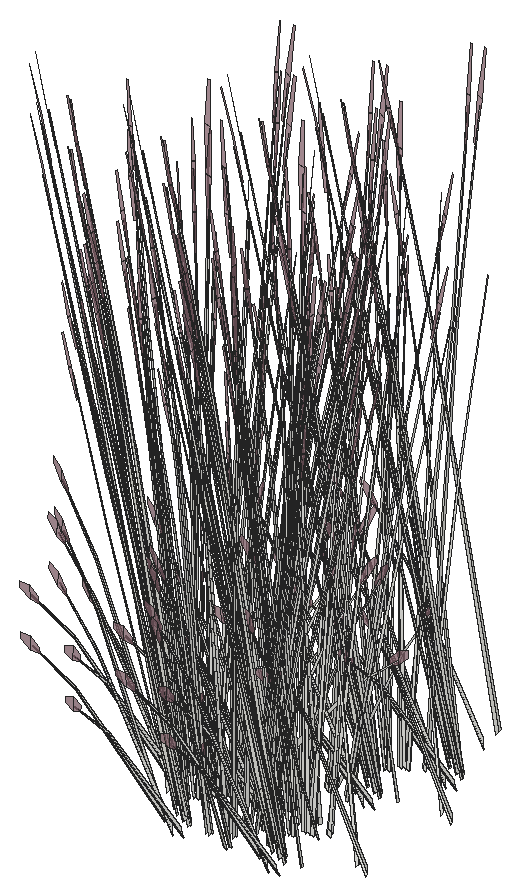
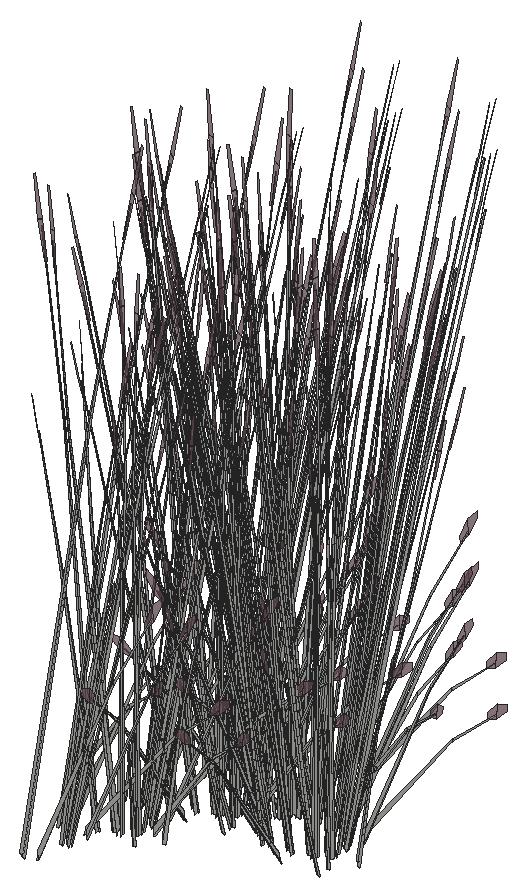
# SketchUp Ruby script. Lengths in inches.
U = 1.inch
M = Sketchup.active_model
def pt(a) = Geom::Point3d.new(a.map { |v| v * U })
def face(e, loops, mat)
  f = e.add_face(loops[0].map { |a| pt(a) })
  loops[1..].each { |l| e.add_face(l.map { |a| pt(a) }).erase! }
  f.material = f.back_material = mat if mat
  f
end
# faces: each face lists its corners as indices into pts; further lists are holes
def faces(e, pts, list, mat = nil) = list.each { |f| face(e, (f[0].is_a?(Array) ? f : [f]).map { |l| l.map { |i| pts[i] } }, mat) }
# xy, xz, yz: faces in a plane at the given z, y or x. An outline is a flat list of corners, or four numbers for a rectangle; further outlines are holes
def ring(l) = l.size == 4 ? [[l[0], l[1]], [l[2], l[1]], [l[2], l[3]], [l[0], l[3]]] : l.each_slice(2).to_a
def flat(e, list, mat, &to3) = list.each { |f| face(e, (f[0].is_a?(Array) ? f : [f]).map { |l| ring(l).map { |u, v| to3.(u, v) } }, mat) }
def xy(e, z, list, mat = nil) = flat(e, list, mat) { |x, y| [x, y, z] }
def xz(e, y, list, mat = nil) = flat(e, list, mat) { |x, z| [x, y, z] }
def yz(e, x, list, mat = nil) = flat(e, list, mat) { |y, z| [x, y, z] }
def lines(e, pts, list) = list.each { |a, b| e.add_line(pt(pts[a]), pt(pts[b])) }
# prism: a flat outline (further loops are holes) pulled along v
def prism(e, loops, v, mat = nil)
  f = face(e, loops, mat); d = Geom::Vector3d.new(v.map { |x| x * U })
  f.pushpull(f.normal.samedirection?(d) ? d.length : -d.length)
end
def box(e, o, s, mat = nil) = prism(e, [[o, [o[0] + s[0], o[1], o[2]], [o[0] + s[0], o[1] + s[1], o[2]], [o[0], o[1] + s[1], o[2]]]], [0, 0, s[2]], mat)
def at(x, y, z, deg = 0) = Geom::Transformation.translation(pt([x, y, z])) * Geom::Transformation.rotation(ORIGIN, Z_AXIS, deg.degrees)
def axes(o, x, y, z) = Geom::Transformation.new([*x, 0, *y, 0, *z, 0, *pt(o).to_a, 1])
def part(name) = M.definitions.add(name)
# library, detail: a bought-in or finely detailed component or shape, given as its bounding box
def library(name, o, s) = part(name).tap { |d| box(d.entities, o, s) }
def detail(e, o, s) = box(e.add_group.entities, o, s)
def put(e, d, t, mat = nil) = e.add_instance(d, t).tap { |i| i.material = mat if mat }
def group(e, t, mat = nil) = e.add_group.tap { |g| g.transformation = t; g.material = mat if mat }.entities
root = M.entities
M.materials.add("LightPink_Translucent").color = [144, 107, 117]
M.materials["LightPink_Translucent"].alpha = 0.75
c1 = part("blade")
p = [[2.15,0.21,22],[0,0.17,0],[0.09,0.45,0],[2.18,0.31,22],[2.29,0.31,22],[0.38,0.45,0],
  [2.48,0.24,33],[2.49,0.24,33],[2.48,0.22,33]]
faces(c1.entities,p,[[0,1,2,3],[4,5,2,3],[6,3,4,7],[8,0,3,6]])
c2 = part("seeds")
p = [[0.3,-0.1,1.38],[-0.01,-0.03,1.59],[-0.01,-0.03,0.03],[0.14,-0.07,-0.07],[0.29,-0.03,3],[0.15,0.01,3.11]]
faces(c2.entities,p,[[0,1,2,3],[1,0,4,5]],"LightPink_Translucent")
c3 = part("blade with seeds")
put(c3.entities,c1,at(0,0,0))
put(c3.entities,c2,axes([2.4,0.25,30.99],[1.5799,-0.05474,1.17369],[-0.12525,1.92788,0.29478],[-0.07173,-0.02425,1.56792]))
put(root,c3,axes([321.88,20.77,52.16],[0.06444,0.01048,1.56736],[0.19934,0.34525,-0.1481],[-0.13191,0.09062,0.27737]))
put(root,c3,axes([323.19,18.85,52.16],[0.03743,0.039,1.56736],[-0.18045,0.35054,-0.1481],[-0.18276,0.00254,0.27737]))
put(root,c3,axes([323.61,18.62,52.17],[-0.10864,-0.00276,1.54581],[-0.34587,0.27582,-0.24447],[-0.18454,-0.05636,0.12397]))
put(root,c3,axes([323.16,20.14,52.18],[0.14265,-0.35629,0.42415],[0.46898,0.12183,0.34973],[-0.18443,0.02141,0.87768]))
put(root,c3,axes([323.13,20.05,52.18],[-0.18545,-0.26643,0.05682],[0.33817,-0.13041,0.44729],[-0.14907,0.02573,0.68204]))
put(root,c3,axes([323.28,21.03,52.18],[-0.12522,-0.35963,0.42415],[0.49122,-0.06241,0.34973],[-0.14477,0.08458,0.87768]))
put(root,c3,axes([323.53,19.24,52.5],[0.41698,-0.28837,0.47505],[0.35962,0.30624,0.3917],[-0.19563,-0.05319,0.983]))
put(root,c3,axes([323.18,20.96,52.18],[-0.34663,-0.16434,0.05682],[0.20181,-0.23402,0.44729],[-0.11113,0.07566,0.68204]))
put(root,c3,axes([323.51,20.15,52.46],[0.41962,0.10901,0.31292],[-0.12239,0.31802,-0.40398],[-0.16894,0.02916,0.77298]))
put(root,c3,axes([323.72,19.24,52.18],[0.02542,-0.29714,0.05682],[0.38391,0.00815,0.44729],[-0.14706,-0.03109,0.68204]))
put(root,c3,axes([322.81,21.78,52.17],[-0.01255,0.07733,1.54581],[0.35618,0.269,-0.24447],[-0.09325,0.12721,0.12397]))
put(root,c3,axes([324.9,18.72,52.8],[-0.33698,0.3746,-0.12034],[-0.48801,-0.21581,-0.66795],[-0.16964,-0.10584,1.01494]))
put(root,c3,axes([323.98,19.46,52.46],[0.28729,0.24465,0.31292],[-0.32804,0.23159,-0.40398],[-0.16667,-0.03524,0.77298]))
put(root,c3,axes([322.58,21.82,52.99],[0.44556,0.1043,-0.05733],[-0.13706,0.32103,-0.25992],[-0.07288,0.04874,0.85731]))
put(root,c3,axes([323.58,20.91,52.46],[0.43951,-0.05584,0.31292],[0.11606,0.31924,-0.40398],[-0.12595,0.08575,0.77298]))
put(root,c3,axes([324.77,17.83,52.16],[-0.00942,0.04684,1.56736],[-0.46458,0.16998,-0.1481],[-0.13671,-0.08689,0.27737]))
put(root,c3,axes([325.82,16.68,52.17],[-0.08245,0.05073,1.54581],[0.00701,0.37067,-0.24447],[-0.18899,0.0482,0.12397]))
put(root,c3,axes([323.99,21.76,52.18],[-0.35954,-0.26661,0.42415],[0.38183,-0.22994,0.34973],[-0.06632,0.12508,0.87768]))
put(root,c3,axes([323.86,21.73,52.18],[-0.41493,-0.01821,0.05682],[0.01138,-0.27493,0.44729],[-0.04342,0.10531,0.68204]))
put(root,c3,axes([324.91,17.06,52.16],[0.06444,0.01048,1.56736],[0.19934,0.34525,-0.1481],[-0.13191,0.09062,0.27737]))
put(root,c3,axes([324.87,19.04,52.46],[0.07798,0.31474,0.31292],[-0.44579,0.08311,-0.40398],[-0.11974,-0.09019,0.77298]))
put(root,c3,axes([322.77,22.57,52.16],[0.05728,-0.02359,1.56736],[0.47345,0.15692,-0.1481],[-0.01113,0.13066,0.27737]))
put(root,c3,axes([326.21,15.14,52.16],[0.03743,0.039,1.56736],[-0.18045,0.35054,-0.1481],[-0.18276,0.00254,0.27737]))
put(root,c3,axes([326.63,14.91,52.17],[-0.10864,-0.00276,1.54581],[-0.34587,0.27582,-0.24447],[-0.18454,-0.05636,0.12397]))
put(root,c3,axes([324.67,18.67,52.5],[0.56246,-0.10044,0.47505],[0.09762,0.39398,0.3917],[-0.13228,-0.11611,0.983]))
put(root,c3,axes([326.18,16.43,52.18],[0.14265,-0.35629,0.42415],[0.46898,0.12183,0.34973],[-0.18443,0.02141,0.87768]))
put(root,c3,axes([326.15,16.34,52.18],[-0.18545,-0.26643,0.05682],[0.33817,-0.13041,0.44729],[-0.14907,0.02573,0.68204]))
put(root,c3,axes([324.8,18.75,52.18],[0.22948,-0.24822,0.05682],[0.32679,0.14452,0.44729],[-0.10565,-0.07958,0.68204]))
put(root,c3,axes([325.3,18.01,52.17],[-0.07723,-0.05479,1.54581],[-0.51538,0.03473,-0.24447],[-0.08225,-0.13104,0.12397]))
put(root,c3,axes([326.3,17.32,52.18],[-0.12522,-0.35963,0.42415],[0.49122,-0.06241,0.34973],[-0.14477,0.08458,0.87768]))
put(root,c3,axes([326.55,15.53,52.5],[0.41698,-0.28837,0.47505],[0.35962,0.30624,0.3917],[-0.19563,-0.05319,0.983]))
put(root,c3,axes([326.2,17.25,52.18],[-0.34663,-0.16434,0.05682],[0.20181,-0.23402,0.44729],[-0.11113,0.07566,0.68204]))
put(root,c3,axes([324.17,21.55,52.46],[0.34164,-0.20573,0.31292],[0.3234,0.23491,-0.40398],[-0.04921,0.11936,0.77298]))
put(root,c3,axes([326.53,16.4375,52.46],[0.41962,0.10901,0.31292],[-0.12239,0.31802,-0.40398],[-0.16894,0.02916,0.77298]))
put(root,c3,axes([323.95,21.6,52.77],[0.55492,0.01936,-0.11927],[-0.01517,0.36657,-0.66198],[-0.03855,0.14118,1.00587]))
put(root,c3,axes([326.74,15.53,52.18],[0.02542,-0.29714,0.05682],[0.38391,0.00815,0.44729],[-0.14706,-0.03109,0.68204]))
put(root,c3,axes([325.84,18.07,52.17],[-0.01255,0.07733,1.54581],[0.35618,0.269,-0.24447],[-0.09325,0.12721,0.12397]))
put(root,c3,axes([327.92,15.02,52.8],[-0.33698,0.3746,-0.12034],[-0.48801,-0.21581,-0.66795],[-0.16964,-0.10584,1.01494]))
put(root,c3,axes([327,15.75,52.46],[0.28729,0.24465,0.31292],[-0.32804,0.23159,-0.40398],[-0.16667,-0.03524,0.77298]))
put(root,c3,axes([325.93,18.99,52.46],[-0.15222,0.30049,0.31292],[-0.44409,-0.08764,-0.40398],[-0.04072,-0.12098,0.77298]))
put(root,c3,axes([325.6,18.11,52.99],[0.44556,0.1043,-0.05733],[-0.13706,0.32103,-0.25992],[-0.07288,0.04874,0.85731]))
put(root,c3,axes([326.6,17.2,52.46],[0.43951,-0.05584,0.31292],[0.11606,0.31924,-0.40398],[-0.12595,0.08575,0.77298]))
put(root,c3,axes([325.125,22.13,52.47],[-0.49753,-0.10215,0.47081],[0.17013,-0.33585,0.3882],[0.0299,0.13207,0.97422]))
put(root,c3,axes([324.99,22.16,52.18],[-0.37205,0.1328,0.05682],[-0.18211,-0.24217,0.44729],[0.03593,0.10675,0.68204]))
put(root,c3,axes([328.62,20.09,52.17],[-0.08245,0.05073,1.54581],[0.00701,0.37067,-0.24447],[-0.18899,0.0482,0.12397]))
put(root,c3,axes([327.79,14.125,52.16],[-0.00942,0.04684,1.56736],[-0.46458,0.16998,-0.1481],[-0.13671,-0.08689,0.27737]))
put(root,c3,axes([327.02,18.05,52.18],[-0.35954,-0.26661,0.42415],[0.38183,-0.22994,0.34973],[-0.06632,0.12508,0.87768]))
put(root,c3,axes([327.7,20.46,52.16],[0.06444,0.01048,1.56736],[0.19934,0.34525,-0.1481],[-0.13191,0.09062,0.27737]))
put(root,c3,axes([326.88,18.02,52.18],[-0.41493,-0.01821,0.05682],[0.01138,-0.27493,0.44729],[-0.04342,0.10531,0.68204]))
put(root,c3,axes([329.01,18.54,52.16],[0.03743,0.039,1.56736],[-0.18045,0.35054,-0.1481],[-0.18276,0.00254,0.27737]))
put(root,c3,axes([327.89,15.33,52.46],[0.07798,0.31474,0.31292],[-0.44579,0.08311,-0.40398],[-0.11974,-0.09019,0.77298]))
put(root,c3,axes([325.8,18.86,52.16],[0.05728,-0.02359,1.56736],[0.47345,0.15692,-0.1481],[-0.01113,0.13066,0.27737]))
put(root,c3,axes([329.43,18.31,52.17],[-0.10864,-0.00276,1.54581],[-0.34587,0.27582,-0.24447],[-0.18454,-0.05636,0.12397]))
put(root,c3,axes([328.98,19.83,52.18],[0.14265,-0.35629,0.42415],[0.46898,0.12183,0.34973],[-0.18443,0.02141,0.87768]))
put(root,c3,axes([326.07,18.71,52.18],[0.37205,-0.1328,0.05682],[0.18211,0.24217,0.44729],[-0.03593,-0.10675,0.68204]))
put(root,c3,axes([324.86,22.73,52.17],[0.064,0.06292,1.54581],[0.51651,0.02472,-0.24447],[0.05194,0.13877,0.12397]))
put(root,c3,axes([328.95,19.74,52.18],[-0.18545,-0.26643,0.05682],[0.33817,-0.13041,0.44729],[-0.14907,0.02573,0.68204]))
put(root,c3,axes([325.94,18.74,52.18],[0.49753,0.10215,0.42415],[-0.17013,0.33585,0.34973],[-0.0299,-0.13207,0.87768]))
put(root,c3,axes([327.69,14.96,52.5],[0.56246,-0.10044,0.47505],[0.09762,0.39398,0.3917],[-0.13228,-0.11611,0.983]))
put(root,c3,axes([325.13,21.88,52.46],[0.15222,-0.30049,0.31292],[0.44409,0.08764,-0.40398],[0.04072,0.12098,0.77298]))
put(root,c3,axes([327.82,15.04,52.18],[0.22948,-0.24822,0.05682],[0.32679,0.14452,0.44729],[-0.10565,-0.07958,0.68204]))
put(root,c3,axes([329.09,20.72,52.18],[-0.12522,-0.35963,0.42415],[0.49122,-0.06241,0.34973],[-0.14477,0.08458,0.87768]))
put(root,c3,axes([329.35,18.93,52.5],[0.41698,-0.28837,0.47505],[0.35962,0.30624,0.3917],[-0.19563,-0.05319,0.983]))
put(root,c3,axes([329,20.65,52.18],[-0.34663,-0.16434,0.05682],[0.20181,-0.23402,0.44729],[-0.11113,0.07566,0.68204]))
put(root,c3,axes([328.32,14.3,52.17],[-0.07723,-0.05479,1.54581],[-0.51538,0.03473,-0.24447],[-0.08225,-0.13104,0.12397]))
put(root,c3,axes([325.73,22.96,52.99],[0.34892,-0.22417,-0.05733],[0.3197,0.24551,-0.25992],[0.02251,0.06957,0.85731]))
put(root,c3,axes([329.33,19.84,52.46],[0.41962,0.10901,0.31292],[-0.12239,0.31802,-0.40398],[-0.16894,0.02916,0.77298]))
put(root,c3,axes([327.19,17.84,52.46],[0.34164,-0.20573,0.31292],[0.3234,0.23491,-0.40398],[-0.04921,0.11936,0.77298]))
put(root,c3,axes([329.54,18.93,52.18],[0.02542,-0.29714,0.05682],[0.38391,0.00815,0.44729],[-0.14706,-0.03109,0.68204]))
put(root,c3,axes([327.5,18.41,52.16],[-0.05128,0.02985,1.56736],[-0.5024,-0.1007,-0.1481],[-0.01819,-0.13025,0.27737]))
put(root,c3,axes([328.63,21.47,52.17],[-0.01255,0.07733,1.54581],[0.35618,0.269,-0.24447],[-0.09325,0.12721,0.12397]))
put(root,c3,axes([330.72,18.42,52.8],[-0.33698,0.3746,-0.12034],[-0.48801,-0.21581,-0.66795],[-0.16964,-0.10584,1.01494]))
put(root,c3,axes([326.98,17.89,52.77],[0.55492,0.01936,-0.11927],[-0.01517,0.36657,-0.66198],[-0.03855,0.14118,1.00587]))
put(root,c3,axes([329.8,19.15,52.46],[0.28729,0.24465,0.31292],[-0.32804,0.23159,-0.40398],[-0.16667,-0.03524,0.77298]))
put(root,c3,axes([326.89,19.32,52.46],[-0.34164,0.20573,0.31292],[-0.3234,-0.23491,-0.40398],[0.04921,-0.11936,0.77298]))
put(root,c3,axes([331.08,24.28,52.17],[-0.08245,0.05073,1.54581],[0.00701,0.37067,-0.24447],[-0.18899,0.0482,0.12397]))
put(root,c3,axes([328.4,21.51,52.99],[0.44556,0.1043,-0.05733],[-0.13706,0.32103,-0.25992],[-0.07288,0.04874,0.85731]))
put(root,c3,axes([326.36,22.05,52.18],[-0.5022,0.08967,0.42415],[-0.08716,-0.35177,0.34973],[0.11811,0.10367,0.87768]))
put(root,c3,axes([329.4,20.6,52.46],[0.43951,-0.05584,0.31292],[0.11606,0.31924,-0.40398],[-0.12595,0.08575,0.77298]))
put(root,c3,axes([326.27,22.12,52.18],[-0.22948,0.24822,0.05682],[-0.32679,-0.14452,0.44729],[0.10565,0.07958,0.68204]))
put(root,c3,axes([330.16,24.66,52.16],[0.06444,0.01048,1.56736],[0.19934,0.34525,-0.1481],[-0.13191,0.09062,0.27737]))
put(root,c3,axes([328.96,15.28,52.46],[-0.15222,0.30049,0.31292],[-0.44409,-0.08764,-0.40398],[-0.04072,-0.12098,0.77298]))
put(root,c3,axes([331.48,16.68,52.17],[-0.08245,0.05073,1.54581],[0.00701,0.37067,-0.24447],[-0.18899,0.0482,0.12397]))
put(root,c3,axes([330.59,17.53,52.16],[-0.00942,0.04684,1.56736],[-0.46458,0.16998,-0.1481],[-0.13671,-0.08689,0.27737]))
put(root,c3,axes([328.14,18.42,52.47],[-0.49753,-0.10215,0.47081],[0.17013,-0.33585,0.3882],[0.0299,0.13207,0.97422]))
put(root,c3,axes([328.01,18.45,52.18],[-0.37205,0.1328,0.05682],[-0.18211,-0.24217,0.44729],[0.03593,0.10675,0.68204]))
put(root,c3,axes([329.8125,21.45,52.18],[-0.35954,-0.26661,0.42415],[0.38183,-0.22994,0.34973],[-0.06632,0.12508,0.87768]))
put(root,c3,axes([331.47,22.74,52.16],[0.03743,0.039,1.56736],[-0.18045,0.35054,-0.1481],[-0.18276,0.00254,0.27737]))
put(root,c3,axes([329.68,21.42,52.18],[-0.41493,-0.01821,0.05682],[0.01138,-0.27493,0.44729],[-0.04342,0.10531,0.68204]))
put(root,c3,axes([330.5625,17.06,52.16],[0.06444,0.01048,1.56736],[0.19934,0.34525,-0.1481],[-0.13191,0.09062,0.27737]))
put(root,c3,axes([331.88,22.51,52.17],[-0.10864,-0.00276,1.54581],[-0.34587,0.27582,-0.24447],[-0.18454,-0.05636,0.12397]))
put(root,c3,axes([326.2,21.83,52.46],[-0.07798,-0.31474,0.31292],[0.44579,-0.08311,-0.40398],[0.11974,0.09019,0.77298]))
put(root,c3,axes([331.4375,24.03,52.18],[0.14265,-0.35629,0.42415],[0.46898,0.12183,0.34973],[-0.18443,0.02141,0.87768]))
put(root,c3,axes([331.4,23.9375,52.18],[-0.18545,-0.26643,0.05682],[0.33817,-0.13041,0.44729],[-0.14907,0.02573,0.68204]))
put(root,c3,axes([330.6875,18.73,52.46],[0.07798,0.31474,0.31292],[-0.44579,0.08311,-0.40398],[-0.11974,-0.09019,0.77298]))
put(root,c3,axes([328.59,22.26,52.16],[0.05728,-0.02359,1.56736],[0.47345,0.15692,-0.1481],[-0.01113,0.13066,0.27737]))
put(root,c3,axes([325.76,22.28,52.16],[0.00149,-0.04731,1.56736],[0.4327,-0.20872,-0.1481],[0.1503,0.0745,0.27737]))
put(root,c3,axes([331.87,15.14,52.16],[0.03743,0.039,1.56736],[-0.18045,0.35054,-0.1481],[-0.18276,0.00254,0.27737]))
put(root,c3,axes([327.2,19.14,52.18],[0.41493,0.01821,0.05682],[-0.01138,0.27493,0.44729],[0.04342,-0.10531,0.68204]))
put(root,c3,axes([327.61,18.69,52.17],[-0.00487,-0.07777,1.54581],[-0.41166,-0.22476,-0.24447],[0.06364,-0.13625,0.12397]))
put(root,c3,axes([327.07,19.11,52.18],[0.35954,0.26661,0.42415],[-0.38183,0.22994,0.34973],[0.06632,-0.12508,0.87768]))
put(root,c3,axes([332.29,14.91,52.17],[-0.10864,-0.00276,1.54581],[-0.34587,0.27582,-0.24447],[-0.18454,-0.05636,0.12397]))
put(root,c3,axes([331.84,16.43,52.18],[0.14265,-0.35629,0.42415],[0.46898,0.12183,0.34973],[-0.18443,0.02141,0.87768]))
put(root,c3,axes([331.55,24.92,52.18],[-0.12522,-0.35963,0.42415],[0.49122,-0.06241,0.34973],[-0.14477,0.08458,0.87768]))
put(root,c3,axes([331.81,16.34,52.18],[-0.18545,-0.26643,0.05682],[0.33817,-0.13041,0.44729],[-0.14907,0.02573,0.68204]))
put(root,c3,axes([330.49,18.36,52.5],[0.56246,-0.10044,0.47505],[0.09762,0.39398,0.3917],[-0.13228,-0.11611,0.983]))
put(root,c3,axes([331.8,23.13,52.5],[0.41698,-0.28837,0.47505],[0.35962,0.30624,0.3917],[-0.19563,-0.05319,0.983]))
put(root,c3,axes([331.45,24.85,52.18],[-0.34663,-0.16434,0.05682],[0.20181,-0.23402,0.44729],[-0.11113,0.07566,0.68204]))
put(root,c3,axes([329.09,15,52.18],[0.37205,-0.1328,0.05682],[0.18211,0.24217,0.44729],[-0.03593,-0.10675,0.68204]))
put(root,c3,axes([327.89,19.03,52.17],[0.064,0.06292,1.54581],[0.51651,0.02472,-0.24447],[0.05194,0.13877,0.12397]))
put(root,c3,axes([330.62,18.44,52.18],[0.22948,-0.24822,0.05682],[0.32679,0.14452,0.44729],[-0.10565,-0.07958,0.68204]))
put(root,c3,axes([328.96,15.03,52.18],[0.49753,0.10215,0.42415],[-0.17013,0.33585,0.34973],[-0.0299,-0.13207,0.87768]))
put(root,c3,axes([327.49,19.96,52.46],[-0.43951,0.05584,0.31292],[-0.11606,-0.31924,-0.40398],[0.12595,-0.08575,0.77298]))
put(root,c3,axes([328.15,18.18,52.46],[0.15222,-0.30049,0.31292],[0.44409,0.08764,-0.40398],[0.04072,0.12098,0.77298]))
put(root,c3,axes([331.95,17.32,52.18],[-0.12522,-0.35963,0.42415],[0.49122,-0.06241,0.34973],[-0.14477,0.08458,0.87768]))
put(root,c3,axes([331.78,24.04,52.46],[0.41962,0.10901,0.31292],[-0.12239,0.31802,-0.40398],[-0.16894,0.02916,0.77298]))
put(root,c3,axes([332.21,15.53,52.5],[0.41698,-0.28837,0.47505],[0.35962,0.30624,0.3917],[-0.19563,-0.05319,0.983]))
put(root,c3,axes([331.86,17.25,52.18],[-0.34663,-0.16434,0.05682],[0.20181,-0.23402,0.44729],[-0.11113,0.07566,0.68204]))
put(root,c3,axes([331.12,17.71,52.17],[-0.07723,-0.05479,1.54581],[-0.51538,0.03473,-0.24447],[-0.08225,-0.13104,0.12397]))
put(root,c3,axes([331.99,23.13,52.18],[0.02542,-0.29714,0.05682],[0.38391,0.00815,0.44729],[-0.14706,-0.03109,0.68204]))
put(root,c3,axes([331.09,25.67,52.17],[-0.01255,0.07733,1.54581],[0.35618,0.269,-0.24447],[-0.09325,0.12721,0.12397]))
put(root,c3,axes([333.18,22.61,52.8],[-0.33698,0.3746,-0.12034],[-0.48801,-0.21581,-0.66795],[-0.16964,-0.10584,1.01494]))
put(root,c3,axes([332.25,23.35,52.46],[0.28729,0.24465,0.31292],[-0.32804,0.23159,-0.40398],[-0.16667,-0.03524,0.77298]))
put(root,c3,axes([329.99,21.24,52.46],[0.34164,-0.20573,0.31292],[0.3234,0.23491,-0.40398],[-0.04921,0.11936,0.77298]))
put(root,c3,axes([332.1875,16.4375,52.46],[0.41962,0.10901,0.31292],[-0.12239,0.31802,-0.40398],[-0.16894,0.02916,0.77298]))
put(root,c3,axes([328.75,19.25,52.99],[0.34892,-0.22417,-0.05733],[0.3197,0.24551,-0.25992],[0.02251,0.06957,0.85731]))
put(root,c3,axes([327.08,21.41,52.46],[-0.28729,-0.24465,0.31292],[0.32804,-0.23159,-0.40398],[0.16667,0.03524,0.77298]))
put(root,c3,axes([332.4,15.53,52.18],[0.02542,-0.29714,0.05682],[0.38391,0.00815,0.44729],[-0.14706,-0.03109,0.68204]))
put(root,c3,axes([331.49,18.07,52.17],[-0.01255,0.07733,1.54581],[0.35618,0.269,-0.24447],[-0.09325,0.12721,0.12397]))
put(root,c3,axes([329.77,21.29,52.77],[0.55492,0.01936,-0.11927],[-0.01517,0.36657,-0.66198],[-0.03855,0.14118,1.00587]))
put(root,c3,axes([327.34,21.63,52.18],[-0.02542,0.29714,0.05682],[-0.38391,-0.00815,0.44729],[0.14706,0.03109,0.68204]))
put(root,c3,axes([333.58,15.02,52.8],[-0.33698,0.3746,-0.12034],[-0.48801,-0.21581,-0.66795],[-0.16964,-0.10584,1.01494]))
put(root,c3,axes([327.38,21.54,52.18],[-0.3723,0.25748,0.42415],[-0.32109,-0.27343,0.34973],[0.17467,0.04749,0.87768]))
put(root,c3,axes([332.66,15.75,52.46],[0.28729,0.24465,0.31292],[-0.32804,0.23159,-0.40398],[-0.16667,-0.03524,0.77298]))
put(root,c3,axes([333.31,26.51,52.16],[0.03743,0.039,1.56736],[-0.18045,0.35054,-0.1481],[-0.18276,0.00254,0.27737]))
put(root,c3,axes([330.53,14.7,52.16],[-0.05128,0.02985,1.56736],[-0.5024,-0.1007,-0.1481],[-0.01819,-0.13025,0.27737]))
put(root,c3,axes([327.56,20.72,52.46],[-0.41962,-0.10901,0.31292],[0.12239,-0.31802,-0.40398],[0.16894,-0.02916,0.77298]))
put(root,c3,axes([330.85,25.71,52.99],[0.44556,0.1043,-0.05733],[-0.13706,0.32103,-0.25992],[-0.07288,0.04874,0.85731]))
put(root,c3,axes([333.73,26.28,52.17],[-0.10864,-0.00276,1.54581],[-0.34587,0.27582,-0.24447],[-0.18454,-0.05636,0.12397]))
put(root,c3,axes([331.85,24.8,52.46],[0.43951,-0.05584,0.31292],[0.11606,0.31924,-0.40398],[-0.12595,0.08575,0.77298]))
put(root,c3,axes([333.28,27.8,52.18],[0.14265,-0.35629,0.42415],[0.46898,0.12183,0.34973],[-0.18443,0.02141,0.87768]))
put(root,c3,axes([329.91,15.62,52.46],[-0.34164,0.20573,0.31292],[-0.3234,-0.23491,-0.40398],[0.04921,-0.11936,0.77298]))
put(root,c3,axes([333.25,27.71,52.18],[-0.18545,-0.26643,0.05682],[0.33817,-0.13041,0.44729],[-0.14907,0.02573,0.68204]))
put(root,c3,axes([327.88,19.91,52.18],[0.34663,0.16434,0.05682],[-0.20181,0.23402,0.44729],[0.11113,-0.07566,0.68204]))
put(root,c3,axes([333.05,21.72,52.16],[-0.00942,0.04684,1.56736],[-0.46458,0.16998,-0.1481],[-0.13671,-0.08689,0.27737]))
put(root,c3,axes([327.79,19.84,52.18],[0.12522,0.35963,0.42415],[-0.49122,0.06241,0.34973],[0.14477,-0.08458,0.87768]))
put(root,c3,axes([331.26,18.11,52.99],[0.44556,0.1043,-0.05733],[-0.13706,0.32103,-0.25992],[-0.07288,0.04874,0.85731]))
put(root,c3,axes([332.27,25.65,52.18],[-0.35954,-0.26661,0.42415],[0.38183,-0.22994,0.34973],[-0.06632,0.12508,0.87768]))
put(root,c3,axes([332.26,17.2,52.46],[0.43951,-0.05584,0.31292],[0.11606,0.31924,-0.40398],[-0.12595,0.08575,0.77298]))
put(root,c3,axes([328.86,19.9,52.16],[-0.06595,-0.00297,1.56736],[-0.27386,-0.31799,-0.1481],[0.10998,-0.10455,0.27737]))
put(root,c3,axes([331.75,18.68,52.46],[-0.15222,0.30049,0.31292],[-0.44409,-0.08764,-0.40398],[-0.04072,-0.12098,0.77298]))
put(root,c3,axes([332.14,25.62,52.18],[-0.41493,-0.01821,0.05682],[0.01138,-0.27493,0.44729],[-0.04342,0.10531,0.68204]))
put(root,c3,axes([329.38,18.34,52.18],[-0.5022,0.08967,0.42415],[-0.08716,-0.35177,0.34973],[0.11811,0.10367,0.87768]))
put(root,c3,axes([333.65,26.9,52.5],[0.41698,-0.28837,0.47505],[0.35962,0.30624,0.3917],[-0.19563,-0.05319,0.983]))
put(root,c3,axes([330.94,21.82,52.47],[-0.49753,-0.10215,0.47081],[0.17013,-0.33585,0.3882],[0.0299,0.13207,0.97422]))
put(root,c3,axes([329.29,18.41,52.18],[-0.22948,0.24822,0.05682],[-0.32679,-0.14452,0.44729],[0.10565,0.07958,0.68204]))
put(root,c3,axes([327.9375,20.82,52.18],[0.18545,0.26643,0.05682],[-0.33817,0.13041,0.44729],[0.14907,-0.02573,0.68204]))
put(root,c3,axes([333.45,14.125,52.16],[-0.00942,0.04684,1.56736],[-0.46458,0.16998,-0.1481],[-0.13671,-0.08689,0.27737]))
put(root,c3,axes([330.81,21.85,52.18],[-0.37205,0.1328,0.05682],[-0.18211,-0.24217,0.44729],[0.03593,0.10675,0.68204]))
put(root,c3,axes([327.9,20.73,52.18],[-0.14265,0.35629,0.42415],[-0.46898,-0.12183,0.34973],[0.18443,-0.02141,0.87768]))
put(root,c3,axes([333.14,22.93,52.46],[0.07798,0.31474,0.31292],[-0.44579,0.08311,-0.40398],[-0.11974,-0.09019,0.77298]))
put(root,c3,axes([332.67,18.05,52.18],[-0.35954,-0.26661,0.42415],[0.38183,-0.22994,0.34973],[-0.06632,0.12508,0.87768]))
put(root,c3,axes([333.625,27.81,52.46],[0.41962,0.10901,0.31292],[-0.12239,0.31802,-0.40398],[-0.16894,0.02916,0.77298]))
put(root,c3,axes([332.54,18.02,52.18],[-0.41493,-0.01821,0.05682],[0.01138,-0.27493,0.44729],[-0.04342,0.10531,0.68204]))
put(root,c3,axes([333.84,26.9,52.18],[0.02542,-0.29714,0.05682],[0.38391,0.00815,0.44729],[-0.14706,-0.03109,0.68204]))
put(root,c3,axes([327.61,21.33,52.17],[0.10831,-0.00661,1.54581],[0.29709,-0.30358,-0.24447],[0.19266,0.04007,0.12397]))
put(root,c3,axes([335.02,26.39,52.8],[-0.33698,0.3746,-0.12034],[-0.48801,-0.21581,-0.66795],[-0.16964,-0.10584,1.01494]))
put(root,c3,axes([329.22,18.125,52.46],[-0.07798,-0.31474,0.31292],[0.44579,-0.08311,-0.40398],[0.11974,0.09019,0.77298]))
put(root,c3,axes([332.94,22.55,52.5],[0.56246,-0.10044,0.47505],[0.09762,0.39398,0.3917],[-0.13228,-0.11611,0.983]))
put(root,c3,axes([333.98,29.47,52.16],[-0.00942,0.04684,1.56736],[-0.46458,0.16998,-0.1481],[-0.13671,-0.08689,0.27737]))
put(root,c3,axes([333.55,15.33,52.46],[0.07798,0.31474,0.31292],[-0.44579,0.08311,-0.40398],[-0.11974,-0.09019,0.77298]))
put(root,c3,axes([334.1,27.12,52.46],[0.28729,0.24465,0.31292],[-0.32804,0.23159,-0.40398],[-0.16667,-0.03524,0.77298]))
put(root,c3,axes([331.45,18.86,52.16],[0.05728,-0.02359,1.56736],[0.47345,0.15692,-0.1481],[-0.01113,0.13066,0.27737]))
put(root,c3,axes([333.07,22.64,52.18],[0.22948,-0.24822,0.05682],[0.32679,0.14452,0.44729],[-0.10565,-0.07958,0.68204]))
put(root,c3,axes([328.78,18.57,52.16],[0.00149,-0.04731,1.56736],[0.4327,-0.20872,-0.1481],[0.1503,0.0745,0.27737]))
put(root,c3,axes([330.22,15.43,52.18],[0.41493,0.01821,0.05682],[-0.01138,0.27493,0.44729],[0.04342,-0.10531,0.68204]))
put(root,c3,axes([330.64,14.98,52.17],[-0.00487,-0.07777,1.54581],[-0.41166,-0.22476,-0.24447],[0.06364,-0.13625,0.12397]))
put(root,c3,axes([330.09,15.4,52.18],[0.35954,0.26661,0.42415],[-0.38183,0.22994,0.34973],[0.06632,-0.12508,0.87768]))
put(root,c3,axes([333.35,14.96,52.5],[0.56246,-0.10044,0.47505],[0.09762,0.39398,0.3917],[-0.13228,-0.11611,0.983]))
put(root,c3,axes([331.89,18.41,52.18],[0.37205,-0.1328,0.05682],[0.18211,0.24217,0.44729],[-0.03593,-0.10675,0.68204]))
put(root,c3,axes([330.68,22.43,52.17],[0.064,0.06292,1.54581],[0.51651,0.02472,-0.24447],[0.05194,0.13877,0.12397]))
put(root,c3,axes([333.57,21.9,52.17],[-0.07723,-0.05479,1.54581],[-0.51538,0.03473,-0.24447],[-0.08225,-0.13104,0.12397]))
put(root,c3,axes([331.76,18.43,52.18],[0.49753,0.10215,0.42415],[-0.17013,0.33585,0.34973],[-0.0299,-0.13207,0.87768]))
put(root,c3,axes([328.74,21.88,52.16],[-0.04566,-0.03421,1.56736],[0.09987,-0.36669,-0.1481],[0.17984,-0.02343,0.27737]))
put(root,c3,axes([333.48,15.04,52.18],[0.22948,-0.24822,0.05682],[0.32679,0.14452,0.44729],[-0.10565,-0.07958,0.68204]))
put(root,c3,axes([330.95,21.58,52.46],[0.15222,-0.30049,0.31292],[0.44409,0.08764,-0.40398],[0.04072,0.12098,0.77298]))
put(root,c3,axes([332.45,25.4375,52.46],[0.34164,-0.20573,0.31292],[0.3234,0.23491,-0.40398],[-0.04921,0.11936,0.77298]))
put(root,c3,axes([330.51,16.25,52.46],[-0.43951,0.05584,0.31292],[-0.11606,-0.31924,-0.40398],[0.12595,-0.08575,0.77298]))
put(root,c3,axes([333.98,14.3,52.17],[-0.07723,-0.05479,1.54581],[-0.51538,0.03473,-0.24447],[-0.08225,-0.13104,0.12397]))
put(root,c3,axes([334.89,25.5,52.16],[-0.00942,0.04684,1.56736],[-0.46458,0.16998,-0.1481],[-0.13671,-0.08689,0.27737]))
put(root,c3,axes([333.88,30.3,52.5],[0.56246,-0.10044,0.47505],[0.09762,0.39398,0.3917],[-0.13228,-0.11611,0.983]))
put(root,c3,axes([332.23,25.49,52.77],[0.55492,0.01936,-0.11927],[-0.01517,0.36657,-0.66198],[-0.03855,0.14118,1.00587]))
put(root,c3,axes([332.85,17.84,52.46],[0.34164,-0.20573,0.31292],[0.3234,0.23491,-0.40398],[-0.04921,0.11936,0.77298]))
put(root,c3,axes([331.54,22.65,52.99],[0.34892,-0.22417,-0.05733],[0.3197,0.24551,-0.25992],[0.02251,0.06957,0.85731]))
put(root,c3,axes([332.63,17.89,52.77],[0.55492,0.01936,-0.11927],[-0.01517,0.36657,-0.66198],[-0.03855,0.14118,1.00587]))
put(root,c3,axes([330.1,17.7,52.46],[-0.28729,-0.24465,0.31292],[0.32804,-0.23159,-0.40398],[0.16667,0.03524,0.77298]))
put(root,c3,axes([333.32,18.1,52.16],[-0.05128,0.02985,1.56736],[-0.5024,-0.1007,-0.1481],[-0.01819,-0.13025,0.27737]))
put(root,c3,axes([334.99,26.7,52.46],[0.07798,0.31474,0.31292],[-0.44579,0.08311,-0.40398],[-0.11974,-0.09019,0.77298]))
put(root,c3,axes([330.37,17.92,52.18],[-0.02542,0.29714,0.05682],[-0.38391,-0.00815,0.44729],[0.14706,0.03109,0.68204]))
put(root,c3,axes([330.4,17.83,52.18],[-0.3723,0.25748,0.42415],[-0.32109,-0.27343,0.34973],[0.17467,0.04749,0.87768]))
put(root,c3,axes([332.71,19.02,52.46],[-0.34164,0.20573,0.31292],[-0.3234,-0.23491,-0.40398],[0.04921,-0.11936,0.77298]))
put(root,c3,axes([330.58,17.01,52.46],[-0.41962,-0.10901,0.31292],[0.12239,-0.31802,-0.40398],[0.16894,-0.02916,0.77298]))
put(root,c3,axes([334.21,22.875,52.46],[-0.15222,0.30049,0.31292],[-0.44409,-0.08764,-0.40398],[-0.04072,-0.12098,0.77298]))
put(root,c3,axes([334.79,26.33,52.5],[0.56246,-0.10044,0.47505],[0.09762,0.39398,0.3917],[-0.13228,-0.11611,0.983]))
put(root,c3,axes([333.4,26.02,52.47],[-0.49753,-0.10215,0.47081],[0.17013,-0.33585,0.3882],[0.0299,0.13207,0.97422]))
put(root,c3,axes([333.27,26.05,52.18],[-0.37205,0.1328,0.05682],[-0.18211,-0.24217,0.44729],[0.03593,0.10675,0.68204]))
put(root,c3,axes([330.91,16.2,52.18],[0.34663,0.16434,0.05682],[-0.20181,0.23402,0.44729],[0.11113,-0.07566,0.68204]))
put(root,c3,axes([334.92,26.41,52.18],[0.22948,-0.24822,0.05682],[0.32679,0.14452,0.44729],[-0.10565,-0.07958,0.68204]))
put(root,c3,axes([330.81,16.13,52.18],[0.12522,0.35963,0.42415],[-0.49122,0.06241,0.34973],[0.14477,-0.08458,0.87768]))
put(root,c3,axes([337.08,16.68,52.17],[-0.08245,0.05073,1.54581],[0.00701,0.37067,-0.24447],[-0.18899,0.0482,0.12397]))
put(root,c3,axes([337.08,22.96,52.17],[-0.08245,0.05073,1.54581],[0.00701,0.37067,-0.24447],[-0.18899,0.0482,0.12397]))
put(root,c3,axes([334.61,15.28,52.46],[-0.15222,0.30049,0.31292],[-0.44409,-0.08764,-0.40398],[-0.04072,-0.12098,0.77298]))
put(root,c3,axes([332.18,21.74,52.18],[-0.5022,0.08967,0.42415],[-0.08716,-0.35177,0.34973],[0.11811,0.10367,0.87768]))
put(root,c3,axes([332.08,21.8125,52.18],[-0.22948,0.24822,0.05682],[-0.32679,-0.14452,0.44729],[0.10565,0.07958,0.68204]))
put(root,c3,axes([333.8,18.42,52.47],[-0.49753,-0.10215,0.47081],[0.17013,-0.33585,0.3882],[0.0299,0.13207,0.97422]))
put(root,c3,axes([335.42,25.68,52.17],[-0.07723,-0.05479,1.54581],[-0.51538,0.03473,-0.24447],[-0.08225,-0.13104,0.12397]))
put(root,c3,axes([331.89,16.1875,52.16],[-0.06595,-0.00297,1.56736],[-0.27386,-0.31799,-0.1481],[0.10998,-0.10455,0.27737]))
put(root,c3,axes([333.67,18.45,52.18],[-0.37205,0.1328,0.05682],[-0.18211,-0.24217,0.44729],[0.03593,0.10675,0.68204]))
put(root,c3,axes([330.96,17.11,52.18],[0.18545,0.26643,0.05682],[-0.33817,0.13041,0.44729],[0.14907,-0.02573,0.68204]))
put(root,c3,axes([336.16,17.06,52.16],[0.06444,0.01048,1.56736],[0.19934,0.34525,-0.1481],[-0.13191,0.09062,0.27737]))
put(root,c3,axes([336.16,23.33,52.16],[0.06444,0.01048,1.56736],[0.19934,0.34525,-0.1481],[-0.13191,0.09062,0.27737]))
put(root,c3,axes([330.92,17.02,52.18],[-0.14265,0.35629,0.42415],[-0.46898,-0.12183,0.34973],[0.18443,-0.02141,0.87768]))
put(root,c3,axes([332.01,21.53,52.46],[-0.07798,-0.31474,0.31292],[0.44579,-0.08311,-0.40398],[0.11974,0.09019,0.77298]))
